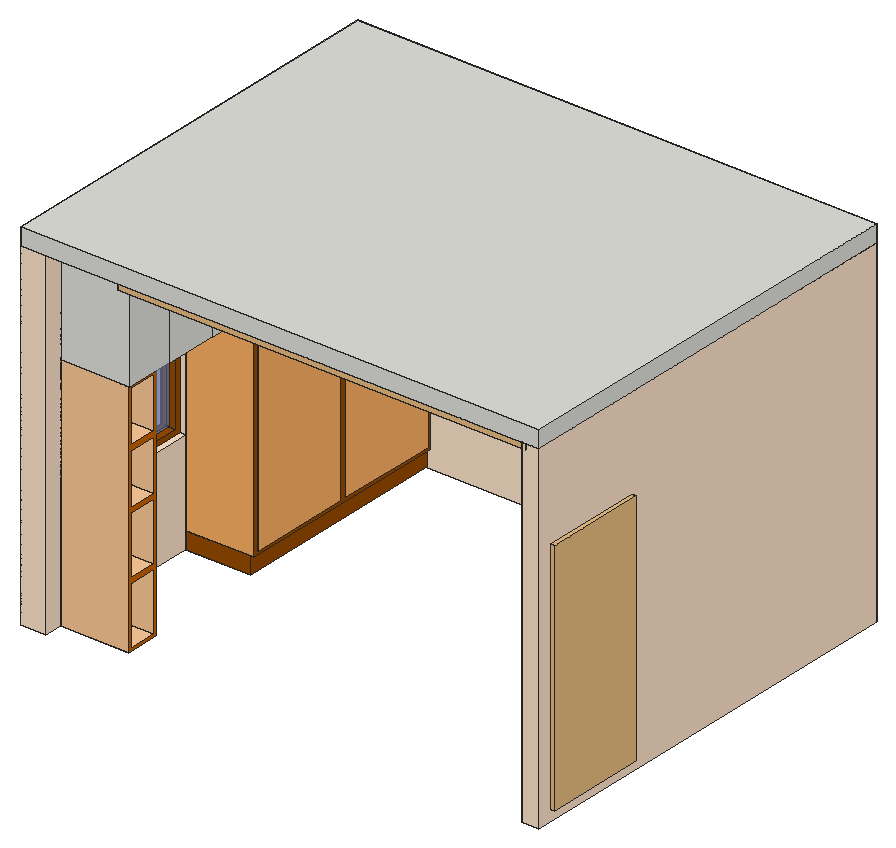
# SketchUp Ruby script. Lengths in millimetres.
U = 1.mm
M = Sketchup.active_model
def pt(a) = Geom::Point3d.new(a.map { |v| v * U })
def face(e, loops, mat)
  f = e.add_face(loops[0].map { |a| pt(a) })
  loops[1..].each { |l| e.add_face(l.map { |a| pt(a) }).erase! }
  f.material = f.back_material = mat if mat
  f
end
# faces: each face lists its corners as indices into pts; further lists are holes
def faces(e, pts, list, mat = nil) = list.each { |f| face(e, (f[0].is_a?(Array) ? f : [f]).map { |l| l.map { |i| pts[i] } }, mat) }
# xy, xz, yz: faces in a plane at the given z, y or x. An outline is a flat list of corners, or four numbers for a rectangle; further outlines are holes
def ring(l) = l.size == 4 ? [[l[0], l[1]], [l[2], l[1]], [l[2], l[3]], [l[0], l[3]]] : l.each_slice(2).to_a
def flat(e, list, mat, &to3) = list.each { |f| face(e, (f[0].is_a?(Array) ? f : [f]).map { |l| ring(l).map { |u, v| to3.(u, v) } }, mat) }
def xy(e, z, list, mat = nil) = flat(e, list, mat) { |x, y| [x, y, z] }
def xz(e, y, list, mat = nil) = flat(e, list, mat) { |x, z| [x, y, z] }
def yz(e, x, list, mat = nil) = flat(e, list, mat) { |y, z| [x, y, z] }
def lines(e, pts, list) = list.each { |a, b| e.add_line(pt(pts[a]), pt(pts[b])) }
# prism: a flat outline (further loops are holes) pulled along v
def prism(e, loops, v, mat = nil)
  f = face(e, loops, mat); d = Geom::Vector3d.new(v.map { |x| x * U })
  f.pushpull(f.normal.samedirection?(d) ? d.length : -d.length)
end
def box(e, o, s, mat = nil) = prism(e, [[o, [o[0] + s[0], o[1], o[2]], [o[0] + s[0], o[1] + s[1], o[2]], [o[0], o[1] + s[1], o[2]]]], [0, 0, s[2]], mat)
def at(x, y, z, deg = 0) = Geom::Transformation.translation(pt([x, y, z])) * Geom::Transformation.rotation(ORIGIN, Z_AXIS, deg.degrees)
def axes(o, x, y, z) = Geom::Transformation.new([*x, 0, *y, 0, *z, 0, *pt(o).to_a, 1])
def part(name) = M.definitions.add(name)
# library, detail: a bought-in or finely detailed component or shape, given as its bounding box
def library(name, o, s) = part(name).tap { |d| box(d.entities, o, s) }
def detail(e, o, s) = box(e.add_group.entities, o, s)
def put(e, d, t, mat = nil) = e.add_instance(d, t).tap { |i| i.material = mat if mat }
def group(e, t, mat = nil) = e.add_group.tap { |g| g.transformation = t; g.material = mat if mat }.entities
root = M.entities
M.materials.add("[Color C01]").color = [255, 229, 204]
M.materials.add("[Color C02]").color = [255, 204, 153]
M.materials.add("[Color C03]").color = [255, 178, 101]
M.materials.add("[Color C06]").color = [204, 102, 0]
M.materials.add("[Color C07]").color = [153, 76, 0]
M.materials.add("[Translucent Glass Sky Reflection]").color = [126, 138, 183]
M.materials["[Translucent Glass Sky Reflection]"].alpha = 0.5
c1 = library("Group\#1",[0,0,0],[3657.6,3368.7,50])
c2 = part("Difference\#1")
xy(c2.entities,0,[[0,0,0,3778.7,4648.2,3778.7,4648.2,0,4495.8,0,4495.8,3538.3,228.6,3538.3,228.6,0]])
xy(c2.entities,100,[[4495.8,123.3,4648.2,1037.3]])
xy(c2.entities,914.4,[[0,310,228.6,1577],[3623.4,3538.3,4343.4,3778.7]])
xy(c2.entities,2133.6,[[0,310,228.6,1577],[3623.4,3538.3,4343.4,3778.7]])
xy(c2.entities,2234,[[4495.8,123.3,4648.2,1037.3]])
xy(c2.entities,3048,[[0,0,228.6,0,228.6,3538.3,4495.8,3538.3,4495.8,0,4648.2,0,4648.2,3778.7,0,3778.7]])
xz(c2.entities,0,[[0,0,228.6,3048],[4495.8,0,4648.2,3048]])
xz(c2.entities,123.3,[[4495.8,100,4648.2,2234]])
xz(c2.entities,310,[[0,914.4,228.6,2133.6]])
xz(c2.entities,1037.3,[[4495.8,100,4648.2,2234]])
xz(c2.entities,1577,[[0,914.4,228.6,2133.6]])
xz(c2.entities,3538.3,[[[228.6,0,4495.8,3048],[3623.4,914.4,4343.4,2133.6]]])
xz(c2.entities,3778.7,[[[0,0,4648.2,3048],[3623.4,914.4,4343.4,2133.6]]])
yz(c2.entities,0,[[[0,0,3778.7,3048],[310,914.4,1577,2133.6]]])
yz(c2.entities,228.6,[[[0,0,3538.3,3048],[310,914.4,1577,2133.6]]])
yz(c2.entities,3623.4,[[3538.3,914.4,3778.7,2133.6]])
yz(c2.entities,4343.4,[[3538.3,914.4,3778.7,2133.6]])
yz(c2.entities,4495.8,[[[0,0,3538.3,3048],[123.3,100,1037.3,2234]]])
yz(c2.entities,4648.2,[[[0,0,3778.7,3048],[123.3,100,1037.3,2234]]])
c3 = library("Group\#8",[0,0,0],[192.3,914,2134])
c4 = part("Difference")
put(c4.entities,c2,at(0,0,0),"[Color C01]")
put(c4.entities,c3,at(4495.8,123.3,100))
p = [[0,3778.7,0],[914.4,3778.7,0],[4343.4,3778.7,0],[3622.7,3778.7,0],[3622.7,3538.3,0],[4343.4,3538.3,0],
  [6429,-5508,0],[6429,-5507.3,0],[5407,-4514.9,0],[5407,-4513.8,0],[10055.2,-5914,0],[10055.2,-6083.7,0],
  [5559,-5771.1,0],[5559,-5771.5,0],[10055.2,-4999.6,0],[9902.8,-4999.6,0],[9902.8,-5914,0]]
lines(root,p,[[0,1],[2,3],[4,5],[6,7],[8,9],[10,11],[12,13],[14,15],[10,16]])
put(root,c1,axes([4528.9,0,3048],[-1,0,0],[0,1,0],[0,0,-1]))
g1 = group(root,at(0,0,3048))
box(g1,[0,0,0],[4648.2,3778.7,152.4])
g2 = group(root,at(40.3,310,914.4),"[Color C07]")
prism(g2,[[[124,1267,1219.2],[124,0,1219.2],[124,0,0],[124,1267,0]],[[124,1224.5,42.5],[124,42.5,42.5],[124,42.5,1176.7],[124,1224.5,1176.7]]],[-124,0,0])
g3 = group(root,at(115,352.5,956.9),"[Translucent Glass Sky Reflection]")
g4 = group(g3,at(-25.4,0,0))
box(g4,[0,0,0],[25.4,1182.1,1134.3])
g5 = group(root,at(3623.4,3594.7,914.4),"[Color C07]")
prism(g5,[[[720,100,1219.2],[720,100,0],[0,100,0],[0,100,1219.2]],[[687.5,100,32.5],[687.5,100,1186.7],[32.5,100,1186.7],[32.5,100,32.5]]],[0,-100,0])
g6 = group(root,at(3655.9,3618.8,946.9),"[Translucent Glass Sky Reflection]")
box(g6,[0,0,0],[655,50.8,1154.2])
put(root,c4,at(0,0,0))
g7 = group(root,at(228.6,1569.8,0))
xy(g7,0,[[0,0,579.6,1968.5]])
xy(g7,152.4,[[0,0,579.6,1968.5],[579.6,0,609.6,1968.5]])
xy(g7,189.3,[[609.6,36.9,619.6,947.3],[609.6,1021.2,619.6,1931.6]])
xy(g7,2096.7,[[609.6,36.9,619.6,947.3],[609.6,1021.2,619.6,1931.6]])
xy(g7,2133.6,[[609.6,0,619.6,482.1],[609.6,492.1,619.6,942.3],[609.6,952.3,619.6,1450.4],[609.6,1460.4,619.6,1968.5]])
xy(g7,3020.4,[[0,0,619.6,0,619.6,482.1,609.6,482.1,609.6,492.1,619.6,492.1,619.6,942.3,609.6,942.3,609.6,952.3,619.6,952.3,619.6,1450.4,609.6,1450.4,609.6,1460.4,619.6,1460.4,619.6,1968.5,0,1968.5]])
xz(g7,0,[[0,152.4,609.6,152.4,609.6,2133.6,619.6,2133.6,619.6,3020.4,0,3020.4]],"[Color C03]")
xz(g7,0,[[0,0,579.6,152.4]],"[Color C07]")
xz(g7,36.9,[[609.6,189.3,619.6,2096.7]])
xz(g7,482.1,[[609.6,2133.6,619.6,3020.4]],"[Color C07]")
xz(g7,492.1,[[609.6,2133.6,619.6,3020.4]],"[Color C07]")
xz(g7,942.3,[[609.6,2133.6,619.6,3020.4]],"[Color C07]")
xz(g7,947.3,[[609.6,189.3,619.6,2096.7]])
xz(g7,952.3,[[609.6,2133.6,619.6,3020.4]],"[Color C07]")
xz(g7,1021.2,[[609.6,189.3,619.6,2096.7]])
xz(g7,1450.4,[[609.6,2133.6,619.6,3020.4]],"[Color C07]")
xz(g7,1460.4,[[609.6,2133.6,619.6,3020.4]],"[Color C07]")
xz(g7,1931.6,[[609.6,189.3,619.6,2096.7]])
xz(g7,1968.5,[[0,152.4,0,3020.4,619.6,3020.4,619.6,2133.6,609.6,2133.6,609.6,152.4]])
xz(g7,1968.5,[[0,0,579.6,152.4]],"[Color C07]")
yz(g7,0,[[0,0,1968.5,152.4],[0,152.4,1968.5,3020.4]])
yz(g7,579.6,[[0,0,1968.5,152.4]],"[Color C07]")
yz(g7,609.6,[[[0,152.4,1968.5,2133.6],[36.9,189.3,947.3,2096.7],[1021.2,189.3,1931.6,2096.7]],[482.1,2133.6,492.1,3020.4],[942.3,2133.6,952.3,3020.4],[1450.4,2133.6,1460.4,3020.4]],"[Color C07]")
yz(g7,619.6,[[0,2133.6,482.1,3020.4],[492.1,2133.6,942.3,3020.4],[952.3,2133.6,1450.4,3020.4],[1460.4,2133.6,1968.5,3020.4]])
yz(g7,619.6,[[36.9,189.3,947.3,2096.7],[1021.2,189.3,1931.6,2096.7]],"[Color C03]")
g8 = group(root,at(228.6,169.7,2135.4))
xy(g8,0,[[0,0,0,1400.2,609.6,1400.2,609.6,1380.5,619.6,1380.5,619.6,928.8,609.6,928.8,609.6,918.8,619.6,918.8,619.6,447.3,609.6,447.3,609.6,437.3,619.6,437.3,619.6,0]],"[Color C03]")
xy(g8,885,[[0,0,619.6,0,619.6,437.3,609.6,437.3,609.6,447.3,619.6,447.3,619.6,918.8,609.6,918.8,609.6,928.8,619.6,928.8,619.6,1380.5,609.6,1380.5,609.6,1400.2,0,1400.2]])
xz(g8,0,[[0,0,619.6,885]])
xz(g8,437.3,[[609.6,0,619.6,885]],"[Color C07]")
xz(g8,447.3,[[609.6,0,619.6,885]],"[Color C07]")
xz(g8,918.8,[[609.6,0,619.6,885]],"[Color C07]")
xz(g8,928.8,[[609.6,0,619.6,885]],"[Color C07]")
xz(g8,1380.5,[[609.6,0,619.6,885]],"[Color C07]")
xz(g8,1400.2,[[0,0,609.6,885]])
yz(g8,0,[[0,0,1400.2,885]])
yz(g8,609.6,[[437.3,0,447.3,885],[918.8,0,928.8,885],[1380.5,0,1400.2,885]],"[Color C07]")
yz(g8,619.6,[[0,0,437.3,885],[447.3,0,918.8,885],[928.8,0,1380.5,885]])
g9 = group(root,at(228.6,169.7,1.8))
xy(g9,0,[[0,0,609.6,304.8]])
xy(g9,21.8,[[369.6,21.8,609.6,283]],"[Color C02]")
xy(g9,543.4,[[369.6,21.8,609.6,283]])
xy(g9,587.1,[[369.6,21.8,609.6,283]],"[Color C02]")
xy(g9,1108.7,[[369.6,21.8,609.6,283]])
xy(g9,1152.4,[[369.6,21.8,609.6,283]],"[Color C02]")
xy(g9,1609.8,[[369.6,21.8,609.6,283]])
xy(g9,1653.5,[[369.6,21.8,609.6,283]],"[Color C02]")
xy(g9,2111.8,[[369.6,21.8,609.6,283]])
xy(g9,2133.6,[[0,0,609.6,304.8]])
xz(g9,0,[[0,0,609.6,2133.6]],"[Color C02]")
xz(g9,21.8,[[369.6,21.8,609.6,543.4],[369.6,587.1,609.6,1108.7],[369.6,1152.4,609.6,1609.8],[369.6,1653.5,609.6,2111.8]])
xz(g9,283,[[369.6,21.8,609.6,543.4],[369.6,587.1,609.6,1108.7],[369.6,1152.4,609.6,1609.8],[369.6,1653.5,609.6,2111.8]],"[Color C02]")
xz(g9,304.8,[[0,0,609.6,2133.6]])
yz(g9,0,[[0,0,304.8,2133.6]])
yz(g9,369.6,[[21.8,21.8,283,543.4],[21.8,587.1,283,1108.7],[21.8,1152.4,283,1609.8],[21.8,1653.5,283,2111.8]],"[Color C02]")
yz(g9,609.6,[[[0,0,304.8,2133.6],[21.8,587.1,283,1108.7],[21.8,21.8,283,543.4],[21.8,1653.5,283,2111.8],[21.8,1152.4,283,1609.8]]],"[Color C06]")
